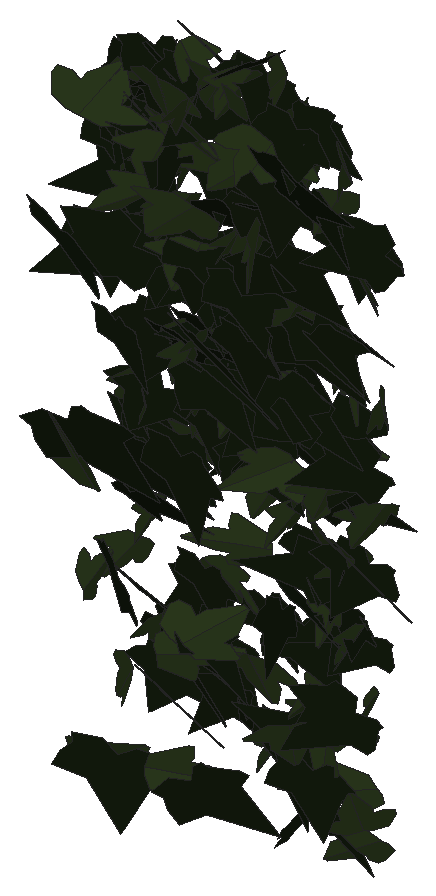
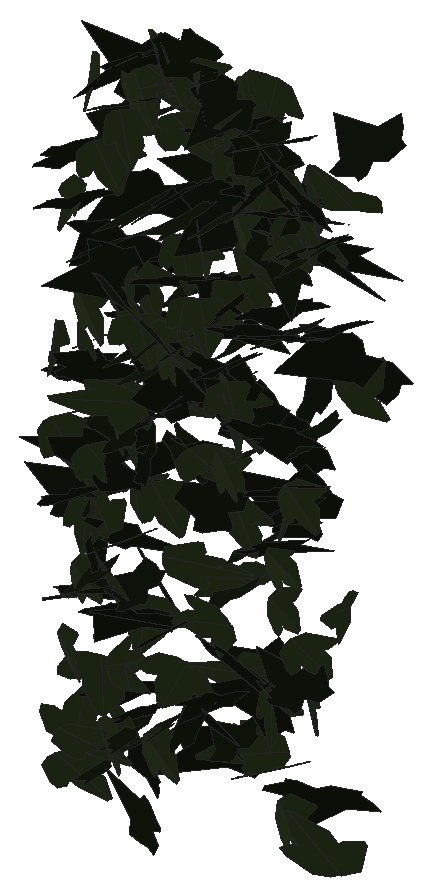
# SketchUp Ruby script. Lengths in millimetres.
U = 1.mm
M = Sketchup.active_model
def pt(a) = Geom::Point3d.new(a.map { |v| v * U })
def face(e, loops, mat)
  f = e.add_face(loops[0].map { |a| pt(a) })
  loops[1..].each { |l| e.add_face(l.map { |a| pt(a) }).erase! }
  f.material = f.back_material = mat if mat
  f
end
# faces: each face lists its corners as indices into pts; further lists are holes
def faces(e, pts, list, mat = nil) = list.each { |f| face(e, (f[0].is_a?(Array) ? f : [f]).map { |l| l.map { |i| pts[i] } }, mat) }
# xy, xz, yz: faces in a plane at the given z, y or x. An outline is a flat list of corners, or four numbers for a rectangle; further outlines are holes
def ring(l) = l.size == 4 ? [[l[0], l[1]], [l[2], l[1]], [l[2], l[3]], [l[0], l[3]]] : l.each_slice(2).to_a
def flat(e, list, mat, &to3) = list.each { |f| face(e, (f[0].is_a?(Array) ? f : [f]).map { |l| ring(l).map { |u, v| to3.(u, v) } }, mat) }
def xy(e, z, list, mat = nil) = flat(e, list, mat) { |x, y| [x, y, z] }
def xz(e, y, list, mat = nil) = flat(e, list, mat) { |x, z| [x, y, z] }
def yz(e, x, list, mat = nil) = flat(e, list, mat) { |y, z| [x, y, z] }
def lines(e, pts, list) = list.each { |a, b| e.add_line(pt(pts[a]), pt(pts[b])) }
# prism: a flat outline (further loops are holes) pulled along v
def prism(e, loops, v, mat = nil)
  f = face(e, loops, mat); d = Geom::Vector3d.new(v.map { |x| x * U })
  f.pushpull(f.normal.samedirection?(d) ? d.length : -d.length)
end
def box(e, o, s, mat = nil) = prism(e, [[o, [o[0] + s[0], o[1], o[2]], [o[0] + s[0], o[1] + s[1], o[2]], [o[0], o[1] + s[1], o[2]]]], [0, 0, s[2]], mat)
def at(x, y, z, deg = 0) = Geom::Transformation.translation(pt([x, y, z])) * Geom::Transformation.rotation(ORIGIN, Z_AXIS, deg.degrees)
def axes(o, x, y, z) = Geom::Transformation.new([*x, 0, *y, 0, *z, 0, *pt(o).to_a, 1])
def part(name) = M.definitions.add(name)
# library, detail: a bought-in or finely detailed component or shape, given as its bounding box
def library(name, o, s) = part(name).tap { |d| box(d.entities, o, s) }
def detail(e, o, s) = box(e.add_group.entities, o, s)
def put(e, d, t, mat = nil) = e.add_instance(d, t).tap { |i| i.material = mat if mat }
def group(e, t, mat = nil) = e.add_group.tap { |g| g.transformation = t; g.material = mat if mat }.entities
root = M.entities
M.materials.add("efeu1").color = [18, 25, 13]
M.materials.add("efeu2").color = [43, 57, 29]
c1 = part("ivyleaf_10")
p = [[0,12.8,-0.8],[-1.5,51.3,-10.9],[-4.9,51,-11.6],[-13.6,26.5,-7.3],[-13.2,15.9,-4.6],[-21.1,19.3,-7.2],
  [-29.5,16.3,-8.3],[-29.2,8.3,-6.2],[-19.7,-9.8,0.5],[-7.6,-13,4],[1,-12.2,5.8],[-0.4,51.1,-11.1],
  [-1.5,51.1,-10.9],[1,-12.4,5.9],[16.9,-12.4,3.5],[35.1,9.1,-5.1],[35,12.9,-6.1],[20.5,16.4,-4.9],
  [15.8,15,-3.8],[15.3,27.6,-7.1],[12.8,31.3,-7.8]]
faces(c1.entities,p,[[0,1,2,3,4,5,6,7,8,9,10],[11,12,0,13,14,15,16,17,18,19,20]],"efeu2")
c2 = part("ivyleaf_9")
p = [[39.1,54.8,31.7],[34.5,51.8,30.2],[-5.3,25.2,17.3],[-17.9,28.3,20.9],[-21.6,21.7,17],[-20.2,4.3,5.3],
  [-22.9,-0.3,2.5],[-17.1,-4,-0.6],[-2,-2.1,-1.2],[-0.7,-15.4,-10.1],[16.6,-22.3,-16.7],[21.1,-15.1,-12.5],
  [32.7,-10.7,-11],[46.1,-1.8,-6.6],[30.8,11.2,3.8]]
faces(c2.entities,p,[[0,1,2,3,4,5,6,7,8,9,10,11,12,13,14]],"efeu1")
put(root,c1,axes([1990.4,834.4,2484],[1.89718,0.20328,-0.47278],[0.77668,0.31566,0.99617],[0.59672,-1.05715,0.20654]))
put(root,c1,axes([2008.6,873.3,2507.4],[0.90197,-0.88313,-0.08799],[0.15661,0.14305,-0.99249],[1.68182,0.46031,0.13961]))
put(root,c1,axes([2017.9,893.5,2124.8],[-0.25535,-0.8722,0.31137],[-0.09813,-0.3071,-0.88245],[1.75985,-0.14368,-0.00403]))
put(root,c1,axes([2023.3,874.5,1919.5],[-0.61177,-0.6764,0.52244],[-0.15273,-0.53181,-0.73791],[1.61941,-0.30568,0.12777]))
put(root,c2,axes([2005.2,850.5,2322.3],[-0.43595,-0.94928,0.0558],[0.05196,-0.06394,-0.97565],[1.80904,-0.22693,0.04147]))
put(root,c2,axes([2002.1,876.3,2441.9],[-0.12544,-0.99389,-0.09302],[0.03031,0.09216,-0.99603],[1.8996,-0.0671,0.00975]))
put(root,c2,axes([1998.1,891.4,2435.3],[0.31687,-0.97049,0.06718],[-0.00048,-0.0682,-0.98459],[1.85145,0.16608,-0.01175]))
put(root,c1,axes([1999.5,851.5,1644.2],[-1.46575,-0.42954,0.52529],[0.97799,0.14972,0.87584],[-0.84338,0.92013,0.1027]))
put(root,c1,axes([2023.9,879.7,2473.3],[0.87061,-0.87487,-0.09808],[0.02962,0.11855,-0.98488],[1.67522,0.45257,0.06839]))
put(root,c1,axes([2030.3,883.7,2462.9],[-0.49832,-0.87203,0.36129],[-0.07538,-0.36445,-0.90837],[1.79487,-0.25741,0.06216]))
put(root,c2,axes([2009,888.6,2495.6],[-0.75426,0.65191,0.63481],[0.61946,-0.54503,0.76291],[1.61719,0.51282,0.00384]))
put(root,c2,axes([2004,869.4,2193.6],[0.43354,-0.91816,0.22903],[0.04855,-0.22953,-0.94553],[1.80033,0.22729,-0.02966]))
put(root,c2,axes([2062,837.9,2413.1],[-1.79112,0.29635,0.29843],[-0.53588,0.09938,-0.98662],[-0.59459,-0.98228,-0.00978]))
put(root,c2,axes([2033.8,890.6,2476.9],[-1.30086,-0.71274,-0.00371],[0.34341,-0.16807,-0.95624],[1.31232,-0.66254,0.24656]))
put(root,c1,axes([2036,775.4,1919.9],[0.06884,0.22167,-0.982],[0.34858,0.96479,0.22453],[1.88399,-0.18661,-0.00566]))
put(root,c1,axes([2040.5,897.6,2036.5],[0.15156,-0.78186,0.49958],[0.09861,-0.49688,-0.78591],[1.76311,0.095,0.00101]))
put(root,c2,axes([2043.4,908.2,2326],[-1.26676,-0.65359,0.21848],[0.05262,-0.32882,-0.89947],[1.31052,-0.61857,0.2473]))
put(root,c2,axes([2014,883,1864.5],[0.09695,-0.55307,0.74732],[0.87473,-0.63561,-0.50172],[1.5381,0.39634,0.23823]))
put(root,c1,axes([2041.3,871.4,2098.6],[0.41269,-0.73874,-0.54662],[0.25339,0.58096,-0.73233],[1.73055,0.09111,0.23758]))
put(root,c2,axes([2061.1,900.8,2045],[-1.21522,-0.36043,0.60223],[-0.77865,-0.47038,-0.71529],[1.08532,-0.74103,0.16112]))
put(root,c2,axes([2017.3,885.9,2479.1],[0.65631,-0.79158,0.49115],[0.34562,-0.45655,-0.86333],[1.73896,0.38949,-0.01378]))
put(root,c1,axes([2045.4,887.4,1971.5],[0.03203,-0.76707,0.51228],[0.19053,-0.50782,-0.76369],[1.74516,0.06952,0.07397]))
put(root,c2,axes([2031.9,889.2,2322.1],[-0.19567,-0.91811,0.24993],[0.13032,-0.25787,-0.91911],[1.80624,-0.08085,0.09339]))
put(root,c2,axes([2050.6,889.6,2118.4],[-1.10863,-0.67175,0.29183],[-0.17403,-0.30325,-0.88057],[1.38299,-0.57664,0.12313]))
put(root,c2,axes([2061.1,867.4,2408.3],[0.01455,0.95187,0.24437],[-0.02998,0.24446,-0.95175],[-1.8701,0.00349,0.01716]))
put(root,c2,axes([2058.3,901.2,2200.5],[-1.45625,-0.54241,-0.20354],[0.30339,0.12705,-0.93784],[1.06003,-0.78151,-0.0112]))
put(root,c1,axes([2046.2,858.1,2425.4],[-0.45595,-0.56106,-0.84043],[0.78634,0.73384,-0.60768],[1.75508,-0.47455,0.05393]))
put(root,c1,axes([2075.3,829.3,2404.7],[-0.39419,-0.47742,0.89381],[-0.66021,-0.82377,-0.52039],[1.81204,-0.40399,0.00484]))
put(root,c2,axes([2056.5,904,1761.5],[-0.77711,-0.71301,0.34579],[-0.06214,-0.37353,-0.80876],[1.50688,-0.38311,0.14497]))
put(root,c1,axes([2061.5,875.1,1839.3],[-0.33324,-0.89884,-0.3085],[0.1594,0.29787,-0.91543],[1.80159,-0.19262,0.02393]))
put(root,c1,axes([2059.9,881.9,2515.6],[-1.87678,0.08208,-0.12222],[0.22115,-0.07435,-0.98746],[-0.17206,-0.99088,0.06397]))
put(root,c2,axes([2043.5,874.2,2093.7],[0.32749,-0.9237,-0.18365],[-0.05822,0.18111,-0.93959],[1.79145,0.17475,0.00304]))
put(root,c2,axes([2043.1,874.3,2423],[0.41327,-0.97144,-0.05633],[-0.01397,0.05608,-0.9954],[1.8519,0.21721,0.00506]))
put(root,c2,axes([2051.3,883.9,2517.2],[0.68377,-0.60975,-0.70099],[-0.545,0.64231,-0.70547],[1.68212,0.45596,0.05637]))
put(root,c2,axes([2078.8,872.8,2538],[-0.14949,0.92193,-0.35814],[0.02584,-0.35823,-0.92513],[-1.88217,-0.07814,0.01575]))
put(root,c2,axes([2092.7,779.1,2363],[-1.75229,-0.44136,0.53496],[-0.92317,-0.22567,-1.02101],[0.94337,-1.04065,-0.00548]))
put(root,c2,axes([2059.4,801.2,1692.5],[-1.22231,-0.76315,-0.42743],[0.55307,0.314,-0.99726],[1.57017,-0.70468,0.01853]))
put(root,c1,axes([2073.8,834.7,1671.4],[0.09971,-1.06977,0.20179],[0.0179,-0.20157,-1.07105],[2.07181,0.05322,-0.00046]))
put(root,c2,axes([2054.1,877.5,2556.8],[0.04618,-0.9734,-0.24861],[0.38565,0.24831,-0.95246],[1.87275,-0.02713,0.20227]))
put(root,c2,axes([2102.9,855.5,2055],[-1.61925,-0.62406,-0.02234],[-0.01204,-0.02913,1.05495],[-1.1884,0.8506,0.01975]))
put(root,c1,axes([2081.8,789.1,1814.8],[0.76927,-0.81495,-0.41775],[-0.14542,0.42502,-0.90308],[1.73684,0.39654,0.10941]))
put(root,c2,axes([2069.8,860.4,2332.2],[-0.66111,-0.96548,-0.06332],[0.02033,0.06345,-1.026],[1.84134,-0.34734,-0.01141]))
put(root,c1,axes([2090.4,840.2,2467.9],[-1.06959,-0.75208,0.30846],[-0.06943,-0.35129,-0.92297],[1.54551,-0.53626,0.17201]))
put(root,c2,axes([2085.4,861.9,2477.2],[-1.27906,-0.71263,-0.16812],[0.28985,0.08717,-0.97825],[1.36304,-0.68726,0.05026]))
put(root,c2,axes([2061.6,875.5,2549.8],[1.20053,-0.76719,0.12365],[0.1526,-0.09415,-0.99322],[1.47107,0.63587,0.00212]))
put(root,c1,axes([2113,883.4,2072],[-1.56425,0.08539,0.49093],[-0.92911,0.05186,-0.82633],[-0.19013,-0.95595,-0.00098]))
put(root,c1,axes([2115.1,669.4,2130.3],[-1.56363,0.69084,-0.51551],[-0.74293,0.33675,1.07342],[1.46266,0.90958,-0.00587]))
put(root,c1,axes([2101.1,879.1,2194.3],[-0.28935,-0.90138,0.25363],[0.0337,-0.25967,-0.91224],[1.78181,-0.14146,0.05844]))
put(root,c2,axes([2088.6,847.1,2472.9],[-1.2723,0.03235,-0.80034],[1.51041,-0.11444,-0.66751],[-0.20646,-1.03651,0.04872]))
put(root,c2,axes([2110.3,881.4,2299],[-1.43614,-0.5788,0.19035],[-0.21425,-0.16534,-0.94902],[1.13964,-0.76046,0.06146]))
put(root,c2,axes([2065.5,875,1835.2],[0.22878,-0.04949,-0.95752],[1.80002,0.16459,0.11023],[0.29966,-0.9509,0.06891]))
put(root,c1,axes([2104,880.7,2441.4],[0.33337,-0.98673,0.0136],[0.00424,-0.01342,-1.00216],[1.87812,0.17518,-0.00015]))
put(root,c1,axes([2108.2,853.6,2393.3],[-0.42325,-0.9539,0.34583],[-0.07592,-0.34555,-0.97876],[1.92959,-0.22283,0.03735]))
put(root,c1,axes([2109.6,892.9,2222],[-0.87174,-0.84692,0.04673],[-0.01001,-0.05027,-0.96265],[1.61428,-0.45767,0.01927]))
put(root,c2,axes([2122.7,895.5,1888.7],[-1.789,0.24426,-0.14113],[0.26206,-0.03125,-0.9712],[-0.46859,-0.95002,-0.00434]))
put(root,c2,axes([2089.1,881.3,2023.3],[0.03855,-0.9087,0.20747],[0.04737,-0.20692,-0.90871],[1.77331,0.02528,0.01976]))
put(root,c2,axes([2064.3,802.2,2043.1],[0.92377,-0.48585,0.89186],[1.26666,-0.5945,-0.68607],[1.46005,0.82315,0.03091]))
put(root,c1,axes([2105,870.6,2571.7],[0.13275,0.97976,0.17504],[0.04632,0.17374,-0.98217],[-1.89363,0.07293,-0.01175]))
put(root,c1,axes([2120.8,889.1,2125.7],[-0.01514,-0.92129,0.17894],[0.02264,-0.17903,-0.92123],[1.78603,-0.00554,0.01319]))
put(root,c2,axes([2079.9,879.4,2191.6],[0.66325,-0.52864,0.7423],[1.16613,-0.45235,-0.60981],[1.28385,0.68398,0.17042]))
put(root,c1,axes([2128,856.5,2505.5],[-0.90195,-0.85715,0.19311],[-0.19386,-0.16433,-0.97939],[1.66094,-0.48464,-0.00945]))
put(root,c1,axes([2124.7,800.8,2568],[-1.78034,0.37737,0.11416],[-0.18974,0.05797,-1.00856],[-0.72598,-0.9406,-0.01635]))
put(root,c2,axes([2090.7,662.7,2430.6],[0.21219,-0.92715,0.85418],[0.53736,-0.81737,-0.92404],[2.33831,0.27197,0.13484]))
put(root,c2,axes([2107.9,900.5,2262.7],[-0.08075,-0.94644,0.00236],[-0.01241,-0.00207,-0.94737],[1.80123,-0.04245,-0.00642]))
put(root,c1,axes([2129.4,851.4,2338.1],[-1.15972,-0.6876,0.3941],[-0.07946,-0.46858,-0.8821],[1.50626,-0.55413,0.2569]))
put(root,c2,axes([2101.3,890.7,1772],[0.25209,-0.68718,0.55852],[0.32494,-0.53432,-0.6979],[1.65373,0.20974,0.05199]))
put(root,c1,axes([2128.6,869,2226.9],[0.05547,-0.97812,-0.05689],[-0.01478,0.05668,-0.97854],[1.86465,0.02955,-0.00607]))
put(root,c2,axes([2118.2,867.8,2551.8],[-0.49765,-0.95649,0.06892],[-0.03932,-0.06581,-0.99158],[1.82468,-0.26228,-0.00257]))
put(root,c2,axes([2093.1,677.4,2182.4],[-0.4277,-0.1748,-1.15039],[1.66549,0.74683,-0.28443],[1.45958,-0.90341,-0.01255]))
put(root,c1,axes([2163.5,821,2488.1],[-0.40892,0.20824,-1.01826],[-1.62576,0.55692,0.29414],[1.12677,0.87912,0.05486]))
put(root,c2,axes([2117.3,876,2589.4],[1.69944,-0.17285,-0.43266],[-0.74142,0.23605,-0.89829],[0.4864,0.96375,0.14242]))
put(root,c1,axes([2156.2,801.2,2419.6],[-1.62966,-0.23854,0.55865],[-0.96449,-0.25182,-0.88428],[0.63741,-0.9909,0.09024]))
put(root,c1,axes([2144.4,846.5,2167.9],[0.29134,-0.90323,-0.35006],[-0.06663,0.34901,-0.91584],[1.84242,0.15545,0.02224]))
put(root,c2,axes([2128.8,849.8,2316.3],[0.72805,-0.53879,-0.81678],[-0.66876,0.74284,-0.65459],[1.73803,0.51153,0.09027]))
put(root,c1,axes([2152.6,896.1,2127.6],[-0.86975,-0.55016,0.61285],[-0.16137,-0.66572,-0.66085],[1.55908,-0.37582,0.27348]))
put(root,c2,axes([2130.9,885.5,2430.7],[-0.15857,-0.90642,0.35778],[-0.00869,-0.35872,-0.90986],[1.8546,-0.07918,0.02633]))
put(root,c1,axes([2114.8,831,1832.6],[0.14989,0.0606,-1.05258],[1.6292,0.6125,0.09932],[1.17138,-0.85964,-0.00344]))
put(root,c2,axes([2106.3,764.8,2110.8],[0.20259,-0.11566,-1.01801],[1.81394,0.38672,0.05572],[0.71547,-0.9477,0.14698]))
put(root,c2,axes([2133.5,879.3,2117.2],[-0.29573,-0.87167,0.31214],[0.15139,-0.3279,-0.8761],[1.75561,-0.11856,0.12812]))
put(root,c2,axes([2111.7,880.4,2212.7],[0.54521,-0.44276,0.83663],[1.01457,-0.64684,-0.52485],[1.48864,0.603,0.05129]))
put(root,c1,axes([2152.9,887.3,2310.8],[-0.70339,-0.89227,-0.08847],[0.04,0.08704,-0.96568],[1.70602,-0.36992,-0.01383]))
put(root,c2,axes([2132.3,885.6,1823],[0.03252,-0.75885,-0.49143],[0.11266,0.4914,-0.75674],[1.71694,-0.01787,0.05896]))
put(root,c2,axes([2135.7,858.2,2347.2],[-0.34331,-0.85108,-0.41918],[0.21039,0.40493,-0.86971],[1.79327,-0.21044,0.02179]))
put(root,c2,axes([2160.7,859.1,2528.3],[-1.49723,-0.55301,0.30356],[-0.18934,-0.37041,-0.93261],[1.18561,-0.75752,0.23441]))
put(root,c2,axes([2184.6,880.5,2240.2],[-1.70886,0.21157,0.39622],[-0.73155,0.09628,-0.92246],[-0.44228,-0.97669,-0.0051]))
put(root,c2,axes([2116.1,893.9,2070.7],[0.91675,-0.5274,0.64224],[0.85492,-0.45931,-0.71408],[1.33068,0.65844,0.01631]))
put(root,c1,axes([2156.8,805.8,2557.5],[-0.00669,-1.0242,-0.09739],[-0.01242,0.09741,-1.02419],[1.95802,-0.00288,-0.00683]))
put(root,c2,axes([2139.5,856.6,1933.2],[0.00744,-0.86888,0.3021],[0.11591,-0.30119,-0.86707],[1.74692,0.02369,0.05624]))
put(root,c1,axes([2131.6,888.3,1918.3],[-0.87044,0.28616,-0.77799],[1.17829,-0.47295,-0.53791],[-1.04911,-0.76861,0.04134]))
put(root,c2,axes([2167.9,871.7,1786],[-1.59614,0.25323,-0.33738],[0.61654,-0.0943,-0.87605],[-0.51424,-0.89905,-0.00314]))
put(root,c1,axes([2176.4,836.8,2568.1],[-1.58597,0.29268,0.4772],[-0.87879,0.12447,-0.88267],[-0.60237,-0.95218,0.0313]))
put(root,c1,axes([2190,878.4,1972.9],[-0.10262,0.07152,0.95533],[-1.26584,-0.69145,0.01423],[1.31223,-0.66141,0.08843]))
put(root,c1,axes([2139.2,787.1,1708.1],[0.12189,0.17176,1.08411],[0.93631,0.96628,-0.18216],[-1.86744,0.49569,-0.02057]))
put(root,c2,axes([2132.1,791,1806.4],[0.63449,-0.69395,0.64405],[0.75338,-0.51809,-0.76314],[1.63682,0.50746,0.1016]))
put(root,c2,axes([2149.1,824.4,2411.9],[1.54928,0.6646,0.32649],[0.45179,0.22536,-1.05062],[-1.33488,0.84762,0.02334]))
put(root,c2,axes([2152.3,842.5,2194.7],[0.53331,-0.88036,-0.34094],[-0.10801,0.33929,-0.92274],[1.79351,0.28221,0.04581]))
put(root,c2,axes([2149.5,866.7,2300.5],[0.90404,-0.83569,-0.09748],[-0.03442,0.10178,-0.96064],[1.60089,0.47411,0.03439]))
put(root,c1,axes([2176.2,863.5,2579],[0.43006,-0.96264,-0.24983],[0.00115,0.25633,-0.98714],[1.89279,0.21856,0.05737]))
put(root,c1,axes([2177.6,883.1,2302.4],[-0.61676,-0.89566,-0.18955],[0.11964,0.17883,-0.95248],[1.73827,-0.3301,-0.0017]))
put(root,c2,axes([2193.4,868.6,2213.6],[-1.50839,0.50214,-0.23003],[0.36477,-0.12729,-0.93823],[-0.98586,-0.81539,0.0048]))
put(root,c1,axes([2188.2,845.2,2382.8],[0.22537,-0.85591,-0.4873],[-0.10658,0.48417,-0.86401],[1.87144,0.13065,0.00948]))
put(root,c1,axes([2192.6,872.4,2373.1],[-0.7325,-0.90588,-0.08156],[0.03349,0.08113,-0.98413],[1.73072,-0.38497,-0.01548]))
put(root,c2,axes([2205.4,862.2,2114.2],[-1.07033,0.81357,-0.37128],[0.4103,-0.30232,-0.98901],[-1.6518,-0.60227,-0.00509]))
put(root,c2,axes([2182.8,887.5,1752.3],[-0.43193,-0.167,0.97727],[-0.17577,-0.99462,-0.19141],[1.87869,-0.13145,0.20678]))
put(root,c1,axes([2197.3,851,2581.1],[-0.45415,-0.88078,0.47831],[-0.00837,-0.49076,-0.90589],[1.90752,-0.21185,0.10991]))
put(root,c1,axes([2222.5,881.8,2251.9],[0.95293,0.03023,-0.87991],[-1.67412,-0.02576,-0.50143],[-0.07108,1.01207,0.01352]))
put(root,c2,axes([2174.9,803.4,1904.6],[0.55864,-1.03921,-0.33354],[-0.17939,0.31996,-1.07986],[2.06944,0.30827,-0.00357]))
put(root,c2,axes([2173.6,885.9,2420.4],[0.64216,-0.92031,-0.08279],[0.0283,0.09354,-0.97914],[1.75839,0.33459,0.04599]))
put(root,c2,axes([2216.6,843.4,2610.4],[-0.47133,0.88747,-0.4298],[-0.00751,-0.44404,-0.91459],[-1.87667,-0.22111,0.11161]))
put(root,c2,axes([2203,901,2340.4],[-1.20693,-0.67483,0.27106],[-0.12608,-0.30454,-0.91317],[1.37831,-0.61877,0.15382]))
put(root,c1,axes([2197,873.4,1828.2],[-1.7691,0.10005,-0.136],[0.25741,-0.01428,-0.93491],[-0.19235,-0.93933,-0.00028]))
put(root,c1,axes([2201.6,847.5,2181.2],[-0.35483,-0.82675,0.56035],[0.16562,-0.5813,-0.82872],[1.8936,-0.10408,0.17748]))
put(root,c2,axes([2179.3,789.3,1707],[0.10467,-0.3085,-1.06393],[0.31219,1.05576,-0.29766],[2.08503,-0.14259,0.09798]))
put(root,c1,axes([2210.3,893.3,2057.6],[-0.73907,-0.86947,0.34539],[-0.089,-0.35546,-0.94739],[1.77833,-0.37914,0.09613]))
put(root,c2,axes([2183.7,874.5,2255.2],[0.78824,-0.81805,-0.35664],[-0.15027,0.35805,-0.91296],[1.69177,0.41295,0.08508]))
put(root,c2,axes([2192,885.5,2173.9],[-0.14918,-0.9477,0.06653],[0.01027,-0.0672,-0.95087],[1.80806,-0.07781,0.01089]))
put(root,c1,axes([2209.9,875.4,2232.3],[-0.1094,-0.96126,0.0887],[-0.01768,-0.0883,-0.96297],[1.83716,-0.05809,-0.00399]))
put(root,c2,axes([2187.7,859.8,2187.8],[0.71705,-0.84763,-0.49417],[-0.35285,0.45831,-0.92748],[1.83372,0.41965,0.01477]))
put(root,c1,axes([2229.9,827.7,2495.1],[-1.27428,-0.43263,0.6152],[-0.73453,-0.5093,-0.7782],[1.22853,-0.75324,0.17283]))
put(root,c2,axes([2194.5,898.5,1892],[0.21677,-0.89327,-0.14883],[-0.03644,0.14759,-0.9005],[1.72312,0.11549,-0.00032]))
put(root,c1,axes([2187.1,773.2,1903],[1.12808,0.36852,-0.87776],[1.26465,0.58028,0.69234],[1.29744,-0.88604,0.08835]))
put(root,c2,axes([2177.7,890.1,2192.5],[1.57189,-0.00109,-0.48629],[0.92543,0.01365,0.82583],[0.01139,-0.95835,0.01231]))
put(root,c1,axes([2216.5,895.4,1735.7],[0.07626,-0.89822,0.35868],[0.0036,-0.35891,-0.89902],[1.84075,0.03791,-0.0131]))
put(root,c2,axes([2194.4,785.4,2231.4],[0.36336,-0.92853,-0.51828],[-0.02495,0.52447,-0.94445],[2.02368,0.17319,0.08142]))
put(root,c1,axes([2235.3,867.3,2219.5],[1.24206,-0.27353,-0.68758],[-1.18024,0.29804,-0.70717],[0.76842,0.89991,0.02522]))
put(root,c2,axes([2203.5,860,2107.4],[-0.03555,-0.69935,-0.72406],[0.09826,0.72256,-0.69924],[1.91334,-0.0501,0.02246]))
put(root,c2,axes([2216.1,873.2,2575.1],[-0.73487,-0.87672,0.31365],[0.11065,-0.36158,-0.93914],[1.76868,-0.34165,0.18907]))
put(root,c2,axes([2207.1,618.3,2052.1],[0.01084,-0.47191,1.12844],[-0.08195,-1.12783,-0.47144],[2.32644,-0.03753,-0.02186]))
put(root,c2,axes([2207.6,849.1,2430],[0.66726,-0.76629,-0.51433],[-0.21107,0.51122,-0.83726],[1.74372,0.35511,0.09547]))
put(root,c2,axes([2213,877.7,1754.6],[0.96703,-0.53307,-0.51418],[-0.34226,0.5161,-0.71276],[1.36741,0.50617,0.18523]))
put(root,c1,axes([2239.7,892.5,2264.4],[-1.19846,-0.72269,0.15139],[-0.03537,-0.18339,-0.95276],[1.40482,-0.62114,0.10516]))
put(root,c2,axes([2219.9,824.5,2338.5],[-0.28186,-0.94071,-0.24912],[0.11354,0.24274,-0.95208],[1.84859,-0.15834,0.02049]))
put(root,c2,axes([2218.5,880,2219.2],[0.85684,-0.79874,-0.27058],[-0.18221,0.25633,-0.91598],[1.59465,0.45847,0.04072]))
put(root,c2,axes([2246.2,842,2162.6],[-1.11041,-0.56341,0.51119],[-0.29165,-0.54397,-0.77445],[1.41819,-0.553,0.24099]))
put(root,c1,axes([2250,848.6,2603.3],[0.66733,-0.78367,-0.54081],[-0.31963,0.51638,-0.85715],[1.78375,0.38571,0.04874]))
put(root,c2,axes([2231.1,884.3,1619.3],[0.13778,0.87428,0.34753],[-0.15973,-0.34116,0.87576],[1.78344,-0.0981,0.05159]))
put(root,c2,axes([2225.3,881.1,2248.6],[0.95924,-0.77526,-0.34102],[-0.27867,0.3111,-0.92365],[1.58763,0.52301,0.04392]))
put(root,c2,axes([2220.2,899.7,2104.9],[0.53877,-0.34009,-0.9045],[1.54465,-0.42787,0.41489],[-0.99817,-0.84568,0.15383]))
put(root,c2,axes([2226.8,705.7,2171.2],[0.04858,-1.21276,0.34059],[-0.00899,-0.34075,-1.21297],[2.39739,0.0233,-0.01145]))
put(root,c1,axes([2249.4,874.8,2039.5],[-0.06038,-0.71298,0.61435],[0.09325,-0.61512,-0.71134],[1.78878,0.008,0.05782]))
put(root,c2,axes([2233,814.7,2271.9],[-0.16821,-0.88095,0.40202],[0.06539,-0.40629,-0.88275],[1.84179,-0.06603,0.06806]))
put(root,c2,axes([2266.8,881.5,1749.4],[-0.40723,-0.90461,-0.2182],[-0.09818,-0.21201,0.92957],[-1.76831,0.2201,-0.00137]))
put(root,c1,axes([2255.6,870.3,2308.3],[-0.27975,-0.94789,0.18202],[-0.00073,-0.18406,-0.95883],[1.83698,-0.14442,0.02734]))
put(root,c2,axes([2281.5,878.8,2286.5],[-0.80652,0.81762,0.32765],[-0.42377,0.25236,-0.9177],[-1.62194,-0.4725,0.07684]))
put(root,c1,axes([2261.1,863.7,2555.3],[-0.10806,-1.01777,-0.0273],[0.00111,0.02731,-1.01936],[1.93772,-0.05677,-0.00094]))
put(root,c2,axes([2237.7,885.4,1709.8],[-0.50384,-0.01634,-0.91051],[1.6795,-0.23873,-0.25229],[-0.42795,-0.91767,0.08185]))
put(root,c2,axes([2253,848.5,1922.5],[-1.1081,0.1107,-0.80949],[1.4203,-0.33256,-0.58224],[-0.63295,-0.94004,0.11065]))
put(root,c2,axes([2233.8,890.7,1928.2],[0.83063,-0.75539,0.27806],[0.31575,-0.2251,-0.8719],[1.49907,0.46597,0.02957]))
put(root,c1,axes([2279.2,815.6,2132.6],[0.93473,0.3893,-0.89438],[-1.31785,-0.56614,-0.62666],[-1.30755,0.8489,-0.00777]))
put(root,c1,axes([2268.7,808.9,2539.3],[2.00204,0.26422,-0.32485],[-0.59629,-0.0861,-1.08459],[-0.52873,1.09758,-0.00688]))
put(root,c2,axes([2302.4,877.5,1973.2],[-1.22653,0.06946,0.66475],[-1.27201,-0.07373,-0.64024],[0.00931,-0.92292,0.10118]))
put(root,c2,axes([2252.3,882.3,1884.7],[-0.32276,-0.69626,-0.56872],[0.53395,0.50886,-0.70663],[1.62554,-0.30539,0.11919]))
put(root,c2,axes([2251.6,886.9,1736.7],[0.85579,-0.75577,-0.17635],[-0.11759,0.1683,-0.87883],[1.47233,0.45273,0.03231]))
put(root,c2,axes([2262.5,907.1,1983.2],[-0.384,-0.86159,0.25274],[-0.00203,-0.25881,-0.88314],[1.70887,-0.19392,0.05574]))
put(root,c2,axes([2257.9,886.3,1888.8],[-0.48526,-0.71747,-0.56983],[0.42658,0.52467,-0.7609],[1.69078,-0.33829,0.02843]))
put(root,c2,axes([2270.3,886.8,2535.8],[-0.84893,-0.85808,0.25092],[0.05799,-0.29484,-0.95413],[1.7005,-0.41832,0.1578]))
put(root,c1,axes([2280.7,869.2,2500],[-0.55596,-0.94657,-0.06972],[0.04241,0.06609,-0.99062],[1.80589,-0.29296,0.0018]))
put(root,c1,axes([2274.3,888.3,1814.2],[0.10075,-0.20072,0.93425],[0.34204,-0.9169,-0.20717],[1.78619,0.1869,-0.01302]))
put(root,c1,axes([2279.4,878.3,2282.2],[1.12948,-0.6578,-0.38916],[-0.12365,0.44751,-0.85549],[1.44935,0.5508,0.23029]))
put(root,c1,axes([2282.4,862.8,2106.5],[0.07288,-1.01028,0.05909],[0.01362,-0.05886,-1.011],[1.92601,0.03864,0.00491]))
put(root,c2,axes([2312.9,814.9,2211.5],[-1.15899,-0.77169,-0.49184],[-0.57007,-0.39015,0.98301],[-1.64567,0.67862,0.00586]))
put(root,c2,axes([2256.9,882.7,2121.6],[0.82518,-0.86162,0.34254],[0.3089,-0.30177,-0.96452],[1.73742,0.46288,0.00879]))
put(root,c1,axes([2299.3,895.3,2078.2],[-0.90472,-0.67383,0.50305],[-0.22345,-0.51903,-0.80617],[1.58471,-0.45788,0.17352]))
put(root,c2,axes([2269.9,837.6,2383.3],[0.89312,-0.83407,-0.32072],[-0.15433,0.32102,-0.95348],[1.69371,0.46907,0.08224]))
put(root,c2,axes([2281.6,809.8,2482.4],[-0.32449,-0.95111,0.35698],[-0.02474,-0.3599,-0.9651],[1.93329,-0.16424,0.04756]))
put(root,c1,axes([2306.6,879.6,1797.3],[-1.91136,-0.14144,0.13334],[-0.24946,-0.02543,-1.01417],[0.2732,-1.01278,0.00685]))
put(root,c2,axes([2273.5,811,2393.9],[-0.31799,-0.45154,-1.02055],[0.70499,0.95098,-0.4814],[2.00352,-0.4063,0.00742]))
put(root,c1,axes([2299.4,833.4,2534.1],[0.2404,-0.97591,0.1992],[0.10989,-0.19328,-0.98354],[1.89246,0.13519,0.03181]))
put(root,c1,axes([2292,887.3,1932.5],[1.24684,-0.70743,0.27215],[0.30355,-0.223,-0.96361],[1.41027,0.67344,-0.0332]))
put(root,c1,axes([2307.7,876.9,2455.3],[-0.85084,-0.83715,0.28329],[-0.07596,-0.29803,-0.94368],[1.68031,-0.43737,0.10079]))
put(root,c2,axes([2268.7,873.8,2309],[1.78453,-0.33755,0.22661],[0.41931,-0.05688,-0.99634],[0.65031,0.96296,0.02058]))
put(root,c1,axes([2305.4,870.2,1711.8],[0.40979,-0.88459,-0.06379],[-0.02964,0.06186,-0.91042],[1.68766,0.21588,-0.0005]))
put(root,c2,axes([2285.7,835.1,2564],[0.5546,-0.61004,-0.77942],[-0.18146,0.79142,-0.65508],[1.87497,0.25704,0.16715]))
put(root,c2,axes([2295.9,822.1,2560.3],[-0.39798,-0.94123,0.33342],[-0.07958,-0.3321,-0.96372],[1.89875,-0.2112,0.02949]))
put(root,c1,axes([2272.7,880,2148.5],[-0.54843,-0.16345,-0.97247],[1.81944,0.20218,-0.31726],[0.46029,-0.99391,0.09539]))
put(root,c1,axes([2331.4,895,1706.3],[-0.7635,-0.01536,0.76306],[-1.12949,-0.53575,-0.32279],[0.91332,-0.6754,0.2387]))
put(root,c1,axes([2295.5,866.6,1748.4],[1.31316,-0.55647,0.39251],[0.55671,-0.2624,-0.88621],[1.17036,0.74918,-0.01885]))
put(root,c1,axes([2287.2,889.8,1994.4],[-0.95896,0.23543,0.8566],[1.3916,-0.4494,0.55361],[0.96024,0.88639,0.05316]))
put(root,c2,axes([2271,676.8,2350.7],[1.27811,-0.97073,0.50529],[0.56679,-0.40836,-1.18033],[2.00419,0.73454,0.01157]))
put(root,c2,axes([2308.9,878.8,1938.8],[0.12854,0.59082,0.71374],[-0.56359,-0.66434,0.57795],[1.67093,-0.26953,0.14003]))
put(root,c2,axes([2275.8,887.7,2075],[0.67585,-0.02501,-0.89925],[1.40612,0.55968,0.27619],[0.97681,-0.78836,0.22461]))
put(root,c2,axes([2348.7,877.8,2166.6],[-0.90039,-0.04164,0.86043],[-1.59419,-0.20693,-0.47057],[0.38273,-0.95986,0.06412]))
put(root,c2,axes([2303,906.1,1919.1],[-0.11725,-0.77135,0.55593],[0.03045,-0.55785,-0.77226],[1.80933,-0.0406,0.04902]))
put(root,c2,axes([2296.7,876.6,1677],[0.77857,-0.80021,-0.12614],[-0.08302,0.11935,-0.89858],[1.53953,0.41112,0.01533]))
put(root,c1,axes([2320.4,780.6,1826.3],[-1.19294,-0.78763,-0.18353],[0.19339,0.15366,-1.00648],[1.52698,-0.63479,-0.01591]))
put(root,c1,axes([2322.3,884.1,1996.2],[-0.61516,-0.84869,-0.22259],[0.18231,0.20166,-0.90799],[1.65987,-0.33668,0.01723]))
put(root,c1,axes([2304.4,735.4,2469],[0.60923,-0.69999,0.92386],[0.99469,-0.76831,-0.76323],[1.969,0.60472,0.09971]))
put(root,c2,axes([2312.5,831.1,1748.4],[-0.53321,-0.89858,-0.19709],[0.16821,0.17879,-0.94075],[1.74274,-0.29219,0.0305]))
put(root,c2,axes([2301.2,820.2,2214.2],[0.72863,-0.74033,-0.48948],[0.01314,0.53555,-0.80461],[1.68907,0.3152,0.21741]))
put(root,c1,axes([2328.7,879.3,2258.2],[0.10781,-0.9507,0.10335],[-0.01757,-0.10407,-0.95226],[1.81995,0.05531,-0.01532]))
put(root,c2,axes([2321.4,881.7,2125.8],[-0.68141,-0.76557,0.37904],[-0.03704,-0.40356,-0.83349],[1.62541,-0.33014,0.13991]))
put(root,c2,axes([2329.7,905.7,1895],[-0.97718,-0.64008,0.39025],[-0.21117,-0.40291,-0.80683],[1.41105,-0.50356,0.14951]))
put(root,c1,axes([2335.5,829.9,2124.3],[-0.71455,-0.88251,0.1429],[-0.042,-0.1458,-0.95836],[1.70094,-0.37433,0.03637]))
put(root,c1,axes([2332.6,881.4,1911.4],[0.14277,-0.81806,0.42556],[0.12826,-0.42096,-0.8211],[1.75031,0.09758,0.02546]))
put(root,c2,axes([2309.8,833.5,2478.3],[0.56363,-0.93341,0.30808],[0.11223,-0.30431,-0.97867],[1.86736,0.30002,-0.03417]))
put(root,c2,axes([2329.2,902.2,2401.2],[-0.61913,-0.91086,0.06434],[0.00515,-0.06926,-0.96686],[1.73786,-0.3243,0.02579]))
put(root,c1,axes([2356.7,876.2,1655.4],[-0.91328,-0.40328,0.5899],[-0.81889,-0.40424,-0.62637],[1.0858,-0.64408,0.02377]))
put(root,c2,axes([2297.9,791,2511.2],[0.56992,-0.45974,1.03584],[1.08966,-0.86323,-0.54865],[1.86136,0.64611,0.00403]))
put(root,c1,axes([2323.5,887.7,2228.9],[0.86571,-0.62548,0.53523],[0.81991,-0.34022,-0.76371],[1.33509,0.61451,0.12196]))
put(root,c2,axes([2319.9,824.7,2317.3],[0.46465,-0.9025,-0.38384],[0.11179,0.4083,-0.92265],[1.86319,0.20057,0.15108]))
put(root,c1,axes([2343.8,894.8,1823.3],[0.51286,-0.86458,0.10976],[0.08348,-0.10129,-0.90552],[1.65657,0.27277,0.01165]))
put(root,c2,axes([2349.6,879.8,2004],[-1.01653,-0.7798,0.21363],[-0.24119,-0.17213,-0.94516],[1.51978,-0.5489,-0.00711]))
put(root,c2,axes([2326.3,813.1,2314],[-0.60753,-0.43545,-0.83254],[0.88937,0.68923,-0.53967],[1.55128,-0.56568,-0.01665]))
put(root,c1,axes([2351.9,831.3,2532.4],[0.5455,-0.72547,-0.63623],[0.17503,0.68123,-0.73534],[1.8281,0.15126,0.26026]))
put(root,c2,axes([2375.2,851.8,2148.5],[-1.2184,-0.42327,0.61702],[-0.99621,-0.32692,-0.76736],[1.0176,-0.82684,-0.01245]))
put(root,c1,axes([2353.2,862.8,2383.7],[-0.96282,0.84599,0.13491],[-0.07431,0.13374,-0.9851],[-1.62873,-0.5062,-0.0348]))
put(root,c1,axes([2362.1,858,1688.6],[-1.0002,-0.72732,-0.37064],[-0.42154,-0.29722,0.8973],[-1.49533,0.57028,-0.00504]))
put(root,c1,axes([2367.1,876.4,2079.3],[-0.61871,-0.92513,0.30258],[-0.15267,-0.29246,-0.98038],[1.84619,-0.33422,0.02033]))
put(root,c2,axes([2376.6,819.3,1850.8],[-1.41242,-0.57989,0.41159],[-0.59204,-0.27023,-0.94162],[1.21703,-0.80445,0.01961]))
put(root,c2,axes([2329.7,873.4,2005.8],[0.70326,-0.7475,0.65713],[0.72311,-0.54193,-0.83011],[1.75076,0.5241,0.07889]))
put(root,c1,axes([2362.6,885.5,2210.1],[0.28567,-0.83511,-0.40447],[0.28573,0.42619,-0.82423],[1.74272,0.06702,0.20144]))
put(root,c2,axes([2385.3,862.2,2417],[-0.97047,-0.35208,0.84626],[-1.13755,-0.60644,-0.61245],[1.3225,-0.77999,0.09419]))
